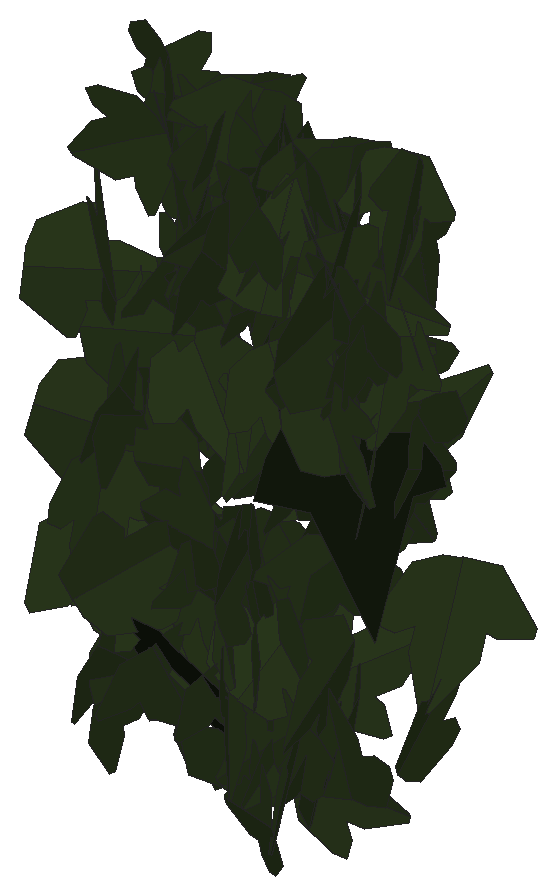
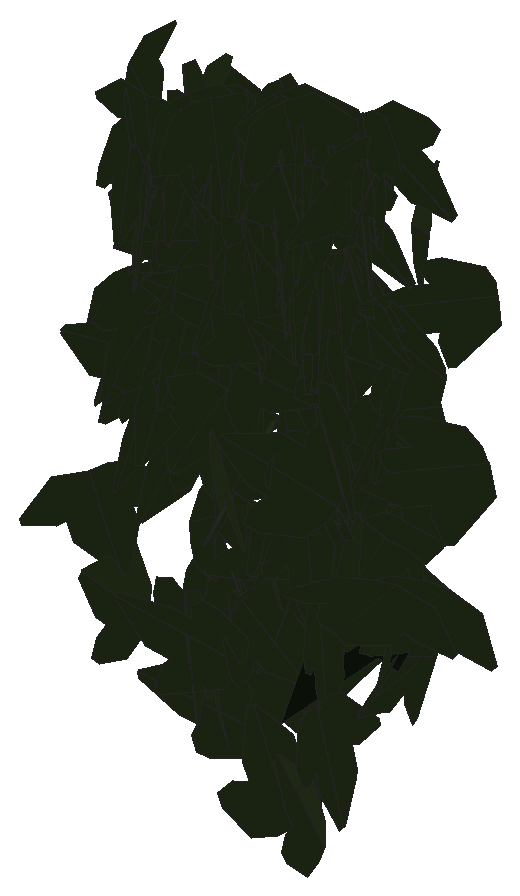
# SketchUp Ruby script. Lengths in inches.
U = 1.inch
M = Sketchup.active_model
def pt(a) = Geom::Point3d.new(a.map { |v| v * U })
def face(e, loops, mat)
  f = e.add_face(loops[0].map { |a| pt(a) })
  loops[1..].each { |l| e.add_face(l.map { |a| pt(a) }).erase! }
  f.material = f.back_material = mat if mat
  f
end
# faces: each face lists its corners as indices into pts; further lists are holes
def faces(e, pts, list, mat = nil) = list.each { |f| face(e, (f[0].is_a?(Array) ? f : [f]).map { |l| l.map { |i| pts[i] } }, mat) }
# xy, xz, yz: faces in a plane at the given z, y or x. An outline is a flat list of corners, or four numbers for a rectangle; further outlines are holes
def ring(l) = l.size == 4 ? [[l[0], l[1]], [l[2], l[1]], [l[2], l[3]], [l[0], l[3]]] : l.each_slice(2).to_a
def flat(e, list, mat, &to3) = list.each { |f| face(e, (f[0].is_a?(Array) ? f : [f]).map { |l| ring(l).map { |u, v| to3.(u, v) } }, mat) }
def xy(e, z, list, mat = nil) = flat(e, list, mat) { |x, y| [x, y, z] }
def xz(e, y, list, mat = nil) = flat(e, list, mat) { |x, z| [x, y, z] }
def yz(e, x, list, mat = nil) = flat(e, list, mat) { |y, z| [x, y, z] }
def lines(e, pts, list) = list.each { |a, b| e.add_line(pt(pts[a]), pt(pts[b])) }
# prism: a flat outline (further loops are holes) pulled along v
def prism(e, loops, v, mat = nil)
  f = face(e, loops, mat); d = Geom::Vector3d.new(v.map { |x| x * U })
  f.pushpull(f.normal.samedirection?(d) ? d.length : -d.length)
end
def box(e, o, s, mat = nil) = prism(e, [[o, [o[0] + s[0], o[1], o[2]], [o[0] + s[0], o[1] + s[1], o[2]], [o[0], o[1] + s[1], o[2]]]], [0, 0, s[2]], mat)
def at(x, y, z, deg = 0) = Geom::Transformation.translation(pt([x, y, z])) * Geom::Transformation.rotation(ORIGIN, Z_AXIS, deg.degrees)
def axes(o, x, y, z) = Geom::Transformation.new([*x, 0, *y, 0, *z, 0, *pt(o).to_a, 1])
def part(name) = M.definitions.add(name)
# library, detail: a bought-in or finely detailed component or shape, given as its bounding box
def library(name, o, s) = part(name).tap { |d| box(d.entities, o, s) }
def detail(e, o, s) = box(e.add_group.entities, o, s)
def put(e, d, t, mat = nil) = e.add_instance(d, t).tap { |i| i.material = mat if mat }
def group(e, t, mat = nil) = e.add_group.tap { |g| g.transformation = t; g.material = mat if mat }.entities
root = M.entities
M.materials.add("efeu1").color = [18, 25, 13]
M.materials.add("efeu2").color = [43, 57, 29]
c1 = part("ivyleaf_10")
p = [[0,0.5,-0.03],[-0.0625,2.02,-0.43],[-0.19,2.01,-0.46],[-0.54,1.05,-0.29],[-0.52,0.625,-0.18],[-0.83,0.76,-0.28],
  [-1.16,0.64,-0.33],[-1.15,0.33,-0.24],[-0.77,-0.39,0.02],[-0.3,-0.51,0.16],[0.04,-0.48,0.23],[-0.02,2.01,-0.4375],
  [-0.06,2.01,-0.43],[0.04,-0.49,0.23],[0.67,-0.49,0.14],[1.38,0.36,-0.2],[1.375,0.51,-0.24],[0.81,0.65,-0.19],
  [0.62,0.59,-0.15],[0.6,1.09,-0.28],[0.5,1.23,-0.31]]
faces(c1.entities,p,[[0,1,2,3,4,5,6,7,8,9,10],[11,12,0,13,14,15,16,17,18,19,20]],"efeu2")
c2 = part("ivyleaf_9")
p = [[1.54,2.16,1.25],[1.36,2.04,1.19],[-0.21,0.99,0.68],[-0.71,1.11,0.82],[-0.85,0.86,0.67],[-0.8,0.17,0.21],
  [-0.9,-0.01,0.1],[-0.67,-0.16,-0.02],[-0.08,-0.08,-0.05],[-0.03,-0.6,-0.4],[0.65,-0.88,-0.66],[0.83,-0.6,-0.49],
  [1.29,-0.42,-0.43],[1.8125,-0.07,-0.26],[1.21,0.44,0.15]]
faces(c2.entities,p,[[0,1,2,3,4,5,6,7,8,9,10,11,12,13,14]],"efeu1")
put(root,c1,axes([512.85,137.88,165.8],[-0.61365,-0.39489,-0.40861],[0.59165,-0.29438,-0.51622],[0.10906,-0.62494,0.50136]))
put(root,c1,axes([512.73,137.47,167.61],[-0.17674,-0.09364,-0.70528],[0.69487,0.13336,-0.19184],[0.15281,-0.71476,0.0566]))
put(root,c1,axes([512.85,137.07,169.74],[-0.01784,-0.10358,-0.65219],[0.5842,0.30172,-0.0639],[0.30789,-0.57848,0.08345]))
put(root,c1,axes([513.58,138.22,171.53],[0.26488,-0.35751,-0.46842],[-0.21107,0.42193,-0.44138],[0.55016,0.334,0.05618]))
put(root,c1,axes([513.83,138.29,171.4],[0.40899,-0.12558,-0.5347],[-0.49938,0.19254,-0.42719],[0.22868,0.64506,0.02342]))
put(root,c1,axes([513.6,138.05,172.16],[0.4583,-0.29069,-0.36046],[-0.16959,0.36655,-0.51122],[0.4309,0.45344,0.18218]))
put(root,c1,axes([513.5,139.38,163.08],[0.33574,-0.55507,0.20984],[-0.08731,0.19227,0.64828],[-0.58695,-0.34611,0.02359]))
put(root,c1,axes([513.97,137.29,171.7],[0.33697,-0.01814,-0.55069],[-0.52119,0.19893,-0.32547],[0.17875,0.6142,0.08915]))
put(root,c1,axes([513.6,138.19,171.47],[-0.35879,0.52593,0.01901],[-0.01059,0.01579,-0.63666],[-0.52617,-0.35895,-0.00015]))
put(root,c1,axes([513.59,137.05,167.17],[0.21935,0.60907,-0.19533],[-0.07898,-0.17912,-0.64723],[-0.63473,0.23277,0.01303]))
put(root,c1,axes([513.98,136.61,170.21],[-0.14496,0.25713,-0.65999],[-0.32484,0.57452,0.29518],[0.62943,0.35572,0.00034]))
put(root,c1,axes([513.66,137.23,168.19],[0.08621,-0.4078,-0.61317],[0.11643,0.61714,-0.39407],[0.72714,-0.05047,0.1358]))
put(root,c1,axes([513.3,138.28,165.88],[-0.64673,-0.45815,-0.35979],[0.61033,-0.38238,-0.49068],[0.10919,-0.57625,0.61165]))
put(root,c1,axes([513.76,137.1875,168.34],[-0.06088,-0.50013,-0.40046],[0.0295,0.39965,-0.5036],[0.64002,-0.066,-0.01488]))
put(root,c1,axes([513.61,138.19,171.77],[-0.03195,-0.32113,-0.5712],[0.25843,0.51935,-0.30643],[0.60216,-0.23993,0.10121]))
put(root,c1,axes([513.75,136.875,164.49],[0.11272,-0.15889,-0.69018],[0.07661,0.6975,-0.14806],[0.70408,-0.05045,0.1266]))
put(root,c1,axes([513.78,136.84,165.15],[-0.03745,-0.42888,-0.50986],[0.0562,0.50681,-0.43044],[0.66388,-0.06709,0.00768]))
put(root,c1,axes([513.86,138.65,164.04],[-0.00588,-0.63791,0.03298],[0.00167,-0.033,-0.63793],[0.63876,-0.00579,0.00197]))
put(root,c1,axes([513.27,137.51,168.89],[0.16767,-0.1235,-0.67754],[0.64533,-0.21538,0.19896],[-0.24054,-0.66391,0.06149]))
put(root,c1,axes([514.35,137.54,167.41],[-0.11672,-0.04175,0.64948],[-0.6326,-0.14775,-0.12318],[0.15291,-0.64313,-0.01386]))
put(root,c1,axes([514.07,138.37,168.32],[0.41892,-0.3409,-0.40351],[-0.26795,0.30669,-0.53728],[0.45524,0.49422,0.05508]))
put(root,c1,axes([514.4,137.75,169.58],[-0.22029,-0.00398,0.66367],[-0.66144,-0.05607,-0.21989],[0.05447,-0.69702,0.0139]))
put(root,c1,axes([514.12,138.47,170.08],[-0.54215,0.29658,0.16266],[-0.17653,0.01404,-0.61399],[-0.28854,-0.56585,0.07002]))
put(root,c1,axes([514.0625,138.02,169.72],[-0.12428,-0.64738,-0.0655],[0.00886,0.065,-0.65919],[0.65062,-0.12454,-0.00354]))
put(root,c1,axes([514.16,138.11,169.99],[-0.16882,-0.60605,-0.25],[0.07234,0.23936,-0.6291],[0.65158,-0.18359,0.00507]))
put(root,c1,axes([513.93,136.68,166.07],[-0.13402,-0.33783,0.67271],[0.23244,0.63133,0.36336],[-0.71599,0.26819,-0.00796]))
put(root,c1,axes([514.28,138.46,171.36],[-0.62156,-0.1435,0.01032],[-0.01151,0.004,-0.63788],[0.14341,-0.62163,-0.00649]))
put(root,c1,axes([514.28,138.13,165.15],[0.10717,-0.62045,-0.16683],[-0.01017,0.16748,-0.62939],[0.64241,0.10616,0.01786]))
put(root,c1,axes([513.91,138.02,168.97],[-0.05865,-0.34172,0.53698],[0.3548,0.43015,0.31248],[-0.52843,0.32674,0.15022]))
put(root,c1,axes([514.36,138.49,170.44],[0.13218,-0.58425,-0.21694],[0.00981,0.22369,-0.59645],[0.62315,0.12041,0.05541]))
put(root,c1,axes([514.38,137.72,170.74],[0.50532,-0.40252,-0.09325],[-0.06531,0.06764,-0.64593],[0.40798,0.50938,0.01209]))
put(root,c1,axes([514.09,138.6,167.28],[-0.13344,-0.43712,0.49629],[0.28939,0.41665,0.44479],[-0.59467,0.30085,0.10509]))
put(root,c1,axes([514.375,137.11,165.08],[-0.27121,-0.5559,-0.2919],[0.13254,0.26012,-0.61851],[0.61373,-0.30183,0.00458]))
put(root,c1,axes([514.33,138.89,162.96],[-0.17352,-0.63394,0.08937],[0.0274,0.08516,0.65725],[-0.63962,0.17563,0.00391]))
put(root,c2,axes([514.18,137.0625,165.29],[0.7452,0.01057,-0.14491],[-0.14507,0.01144,-0.74516],[-0.00819,0.75908,0.01325]))
put(root,c1,axes([514.4,137.58,171.39],[-0.21766,0.6227,0.01951],[-0.00888,0.01756,-0.65964],[-0.62294,-0.21783,0.00259]))
put(root,c1,axes([514.13,137.29,165.84],[0.54414,0.22993,0.3502],[0.31112,0.16265,-0.5902],[-0.28056,0.62631,0.02471]))
put(root,c1,axes([514.5,137.49,166.12],[-0.56081,0.34214,-0.00262],[0.00161,-0.00238,-0.65694],[-0.34214,-0.56081,0.00119]))
put(root,c1,axes([514.53,138.13,171.75],[0.19232,-0.6045,-0.13853],[0.03492,0.15536,-0.62948],[0.61919,0.179,0.07853]))
put(root,c1,axes([514.52,138.26,167.42],[-0.05116,-0.50073,-0.41595],[0.0861,0.40837,-0.50219],[0.64524,-0.09419,0.03403]))
put(root,c1,axes([515.03,137.06,166.9],[-0.08013,0.00077,0.65378],[-0.65112,0.05918,-0.07987],[-0.05883,-0.656,-0.00643]))
put(root,c1,axes([514.48,137.93,171.34],[0.07676,-0.47822,0.43051],[0.21187,-0.3906,-0.47166],[0.60757,0.19663,0.11009]))
put(root,c1,axes([514.69,138.3,172.05],[-0.30495,-0.55748,0.12489],[0.00644,-0.14492,-0.63113],[0.57126,-0.29596,0.07379]))
put(root,c1,axes([514.56,138.44,171.42],[0.38938,-0.48932,0.14193],[0.08873,-0.11077,-0.62534],[0.5017,0.39936,0.00045]))
put(root,c1,axes([514.72,138.41,170.64],[0.25734,-0.56848,-0.14836],[-0.00045,0.16178,-0.62067],[0.58752,0.24912,0.0645]))
put(root,c1,axes([514.92,138.125,172.03],[-0.41926,-0.40959,0.25796],[-0.07906,-0.27875,-0.57109],[0.47756,-0.40574,0.13193]))
put(root,c1,axes([514.86,137.73,166.19],[-0.22876,-0.6235,-0.0101],[0.00452,0.0091,-0.66414],[0.62356,-0.22881,0.00111]))
put(root,c1,axes([515.07,138.4375,171.2],[-0.16129,-0.60038,0.14721],[-0.01655,-0.14788,-0.62129],[0.61794,-0.16067,0.02178]))
put(root,c1,axes([514.6875,137.42,168.93],[0.52805,0.24001,0.31496],[0.28358,0.1372,-0.58],[-0.27638,0.59934,0.00665]))
put(root,c1,axes([515.01,138.02,171.85],[-0.03878,0.49339,0.40523],[-0.10112,0.3961,-0.49196],[-0.63041,-0.09389,0.05398]))
put(root,c1,axes([515.14,138.46,170.15],[-0.02485,-0.6374,-0.01661],[-0.00182,0.01669,-0.63788],[0.63762,-0.0248,-0.00246]))
put(root,c1,axes([515.125,137.73,170.91],[-0.05733,0.00792,-0.69212],[-0.17006,-0.67336,0.00639],[-0.67095,0.17,0.05752]))
put(root,c1,axes([515.09,137.49,166.67],[-0.4488,-0.41114,-0.31279],[0.22186,0.22078,-0.60854],[0.46653,-0.50051,-0.0115]))
put(root,c1,axes([514.73,137.41,166.33],[0.45052,-0.16717,0.56701],[0.54609,-0.15526,-0.47968],[0.22633,0.70736,0.02871]))
put(root,c1,axes([515.23,138.33,171.35],[0.03482,-0.62539,-0.12878],[0.0028,0.12912,-0.62629],[0.63851,0.03354,0.00977]))
put(root,c1,axes([515.24,138.1,171.66],[0.18577,-0.58758,-0.16925],[0.00891,0.17947,-0.61328],[0.6114,0.17591,0.06036]))
put(root,c1,axes([515.27,138.22,164.91],[-0.14679,-0.50179,0.37147],[0.0513,-0.39,-0.50655],[0.62221,-0.08622,0.1294]))
put(root,c1,axes([515.14,137.63,166.29],[-0.61598,0.16189,0.30669],[0.29357,-0.08938,0.63681],[0.18462,0.68228,0.01065]))
put(root,c1,axes([515.25,137.21,165.14],[-0.21552,-0.48565,-0.40585],[0.18304,0.36258,-0.53108],[0.60586,-0.2823,0.01608]))
put(root,c1,axes([515.3,138.2,168.33],[-0.16799,-0.36698,0.51188],[0.11684,-0.53874,-0.34789],[0.61891,0.0021,0.20462]))
put(root,c1,axes([515.375,137.79,170.16],[0.03622,-0.59354,-0.25176],[0.02959,0.25342,-0.5932],[0.64405,0.02174,0.04141]))
put(root,c1,axes([515.42,136.65,170.94],[-0.00724,-0.47935,-0.49437],[0.03839,0.49334,-0.47892],[0.68753,-0.03259,0.02154]))
put(root,c1,axes([515.19,137.54,163.7],[-0.42781,-0.42933,0.34425],[0.26159,0.22496,0.60565],[-0.48415,0.50092,0.02305]))
put(root,c1,axes([515.53,137.92,169.53],[0.20746,-0.57715,-0.18427],[-0.03543,0.18289,-0.61269],[0.60482,0.20868,0.02732]))
put(root,c1,axes([515.82,137.01,171.4],[-0.47564,0.162,0.39647],[-0.41372,-0.02057,-0.48794],[-0.11076,-0.61887,0.12]))
put(root,c1,axes([515.54,137.4,169],[0.26815,-0.36345,0.57601],[-0.23798,0.53003,0.44522],[-0.63816,-0.35037,0.076]))
put(root,c1,axes([515.32,137.25,165.11],[-0.15294,0.53976,-0.39567],[0.11258,-0.37934,-0.56099],[-0.65971,-0.18986,-0.00401]))
put(root,c1,axes([515.96,137.07,163.53],[-0.1417,0.05142,0.62374],[-0.59714,0.18037,-0.15053],[-0.18738,-0.61367,0.00802]))
put(root,c1,axes([515.78,136.6,166.65],[-0.00549,-0.01778,0.68873],[-0.4264,0.54108,0.01057],[-0.54116,-0.42616,-0.01531]))
put(root,c1,axes([516.03,137.43,164.55],[-0.45792,-0.06403,0.53508],[-0.51627,-0.14922,-0.45968],[0.15452,-0.68828,0.04988]))
put(root,c1,axes([515.3,137.75,165.53],[0.0449,-0.11336,0.64522],[0.48975,-0.42372,-0.10853],[0.43509,0.48865,0.05557]))
put(root,c1,axes([515.78,137.93,171.69],[-0.53871,0.31995,0.11542],[-0.12896,0.00792,-0.62386],[-0.31474,-0.55088,0.05806]))
put(root,c1,axes([515.4,137.7,169.84],[0.33476,-0.3555,-0.47492],[0.33213,-0.33953,0.48826],[-0.49155,-0.47152,0.00647]))
put(root,c1,axes([515.79,137.99,164.39],[0.07036,0.32415,-0.55107],[-0.11991,-0.53787,-0.3317],[-0.628,0.13902,0.00159]))
put(root,c1,axes([516.11,137.59,169.7],[0.50092,0.00863,0.51223],[-0.50939,0.08467,0.49672],[-0.05455,-0.71143,0.06533]))
put(root,c1,axes([515.83,137.88,169.6],[0.04992,-0.38401,-0.51185],[0.06174,0.5139,-0.37953],[0.6369,-0.01972,0.07691]))
put(root,c1,axes([515.33,138.34,169.2],[-0.07088,-0.19303,0.65615],[0.60537,0.28929,0.1505],[-0.3183,0.59318,0.14012]))
put(root,c1,axes([515.83,137.63,170.7],[-0.20664,-0.53988,-0.30294],[0.13466,0.27252,-0.57753],[0.60424,-0.24536,0.02511]))
put(root,c1,axes([515.93,138.25,171.65],[-0.39204,-0.51318,0.08154],[0.03388,-0.12718,-0.63748],[0.51851,-0.3797,0.10331]))
put(root,c1,axes([515.91,138.0625,166.99],[0.22098,-0.60664,-0.00253],[-0.00087,0.00238,-0.64563],[0.60665,0.22098,-0.00001]))
put(root,c1,axes([515.78,137.29,170.42],[0.49325,0.3722,-0.16877],[0.13694,0.09872,0.61791],[0.38506,-0.51189,-0.00355]))
put(root,c1,axes([515.66,137.25,165.28],[0.5017,0.21544,-0.38775],[0.32517,0.21954,0.54271],[0.30171,-0.59486,0.05986]))
put(root,c1,axes([516.05,137.99,164.1875],[0.15354,-0.61507,-0.08584],[-0.0151,0.0847,-0.63392],[0.62085,0.15417,0.00581]))
put(root,c1,axes([515.54,138.73,164.57],[0.32504,0.02522,-0.59187],[0.57766,0.1362,0.32304],[0.13135,-0.66137,0.04396]))
put(root,c1,axes([516.1,137.21,166.46],[0.31977,-0.19965,-0.61096],[0.00723,0.68347,-0.21956],[0.64272,0.09165,0.30644]))
put(root,c1,axes([516.18,138.3,171.65],[-0.25248,-0.59193,0.08358],[0.01803,-0.09823,-0.64121],[0.59753,-0.24715,0.05466]))
put(root,c1,axes([515.87,138.23,167.75],[0.45126,0.33707,0.3113],[0.25941,0.17273,-0.56306],[-0.37846,0.5203,-0.01475]))
put(root,c1,axes([516.27,138.23,164.58],[0.22996,-0.53729,-0.27231],[-0.08288,0.26049,-0.58395],[0.59663,0.24327,0.02384]))
put(root,c1,axes([516.27,137.49,168.16],[-0.01388,-0.57456,-0.32341],[0.00142,0.32345,-0.5747],[0.65933,-0.01279,-0.00557]))
put(root,c1,axes([515.72,138.23,163.44],[-0.05873,-0.04999,0.68185],[0.66965,0.13374,0.06749],[-0.13781,0.67118,0.03734]))
put(root,c1,axes([516.14,137.375,164.67],[0.4345,-0.46873,0.30165],[0.20045,-0.22549,-0.63911],[0.52011,0.47847,-0.00569]))
put(root,c1,axes([516.19,137.59,169.34],[0.01159,-0.16452,-0.62767],[0.02812,-0.62705,0.16488],[-0.64826,-0.03014,-0.00407]))
put(root,c1,axes([516.41,137.57,169.34],[-0.02473,0.03408,0.67814],[-0.22507,0.63981,-0.04036],[-0.64061,-0.2261,-0.01199]))
put(root,c1,axes([516.17,136.98,169.54],[0.36435,0.51118,0.17961],[0.0816,0.1622,-0.62718],[-0.53564,0.37242,0.02663]))
put(root,c1,axes([516.44,137.64,166.9],[-0.24329,-0.56355,0.17761],[0.00176,-0.19277,-0.60923],[0.59088,-0.23147,0.07494]))
put(root,c1,axes([516.36,137.98,168.77],[-0.14984,-0.53214,-0.32558],[0.14705,0.29527,-0.55029],[0.60626,-0.20314,0.05301]))
put(root,c1,axes([516.46,138.03,170.99],[-0.56623,0.29359,-0.00032],[0.00048,0.00023,-0.63782],[-0.29359,-0.56623,-0.00042]))
put(root,c1,axes([516.58,137.71,164.01],[-0.66682,-0.09016,-0.06399],[-0.06233,-0.01655,0.67284],[-0.09131,0.66968,0.00801]))
put(root,c1,axes([516.5,138.3,168.26],[-0.27107,-0.58819,-0.26203],[0.13452,0.22631,-0.64715],[0.62971,-0.30154,0.02544]))
put(root,c1,axes([516.28,137.37,169.55],[0.04361,-0.11778,0.71708],[0.37618,0.61829,0.07868],[-0.62175,0.36583,0.0979]))
put(root,c1,axes([516.53,137.6,165.58],[0.02746,-0.20104,0.6447],[0.27965,-0.58393,-0.194],[0.6147,0.27464,0.05946]))
put(root,c1,axes([516.76,137.65,171.55],[0.2716,-0.55572,-0.21183],[-0.04667,0.21224,-0.61663],[0.59289,0.27128,0.04849]))
put(root,c1,axes([516.65,138.5,168.99],[-0.29508,-0.48275,-0.34445],[0.20228,0.27973,-0.56533],[0.55747,-0.35703,0.02281]))
put(root,c1,axes([517.11,136.89,170.86],[-0.09071,0.19805,-0.6082],[-0.41302,0.45091,0.20843],[0.4884,0.4181,0.0633]))
put(root,c1,axes([516.71,137.69,166.91],[-0.25282,-0.46382,-0.38639],[0.17549,0.34435,-0.52818],[0.5776,-0.30763,-0.00865]))
put(root,c1,axes([516.78,138.33,167.67],[0.01121,-0.53491,-0.37796],[0.12939,0.37237,-0.52317],[0.64206,-0.0657,0.11203]))
put(root,c1,axes([516.93,137.6,168.35],[0.42317,-0.44683,-0.21759],[-0.13813,0.16877,-0.61523],[0.47741,0.4449,0.01486]))
put(root,c1,axes([516.93,137.08,168.83],[0.03239,0.65673,-0.17983],[-0.00395,0.18021,0.65741],[0.68089,-0.03019,0.01236]))
put(root,c1,axes([516.98,136.4,170.27],[0.08915,-0.12975,0.77518],[-0.26672,0.72886,0.15267],[-0.73933,-0.27859,0.03839]))
put(root,c1,axes([517.13,138.14,170.3125],[-0.3309,0.32557,0.43627],[-0.33746,0.27793,-0.46336],[-0.42714,-0.47179,0.0281]))
put(root,c1,axes([517.27,137.16,170.625],[-0.52627,-0.00248,0.43532],[-0.43531,0.00979,-0.52619],[-0.00433,-0.68291,-0.00912]))
put(root,c1,axes([516.71,137.1,169.23],[-0.53467,0.16729,-0.30873],[0.29059,-0.10493,-0.56011],[-0.19713,-0.60842,0.01171]))
put(root,c1,axes([516.77,138.43,171.64],[0.62939,0.04433,0.095],[0.09595,-0.01054,-0.63072],[-0.04225,0.63644,-0.01706]))
put(root,c1,axes([517.02,137.5,169.96],[-0.00918,-0.54484,-0.35414],[0.08233,0.35035,-0.54114],[0.64459,-0.05251,0.06407]))
put(root,c1,axes([516.54,137.43,170.58],[0.13342,0.0934,0.70297],[0.53369,0.4578,-0.16212],[-0.46697,0.54989,0.01557]))
put(root,c1,axes([516.76,138.29,168.12],[0.21058,0.25817,-0.65257],[0.40139,0.51456,0.3331],[0.57566,-0.45323,0.00646]))
put(root,c1,axes([517.08,138.36,171.06],[-0.04769,-0.61268,-0.18724],[0.0886,0.17965,-0.6104],[0.6345,-0.07114,0.07116]))
put(root,c1,axes([517.24,138.18,168.76],[-0.25429,-0.62194,0.03039],[-0.01117,-0.02826,-0.67192],[0.62258,-0.25453,0.00035]))
put(root,c2,axes([516.92,137.48,168.72],[-0.08579,-0.76793,-0.21996],[0.04423,0.21632,-0.77247],[0.79759,-0.0946,0.01918]))
put(root,c1,axes([517.2,138.29,164.39],[0.20728,-0.47978,0.46203],[-0.15792,0.43469,0.52224],[-0.64709,-0.25977,0.02055]))
put(root,c1,axes([517.1,137.84,169.9],[0.64732,-0.0105,0.03973],[0.03978,0.00237,-0.64739],[0.01033,0.64853,0.003]))
put(root,c1,axes([517.19,137.43,170.24],[0.06673,-0.4912,-0.42817],[0.09597,0.43312,-0.48192],[0.64451,-0.01363,0.11609]))
put(root,c1,axes([517.42,137.92,168.32],[0.05905,-0.33084,-0.56657],[-0.00445,0.56865,-0.33252],[0.65608,0.03363,0.04874]))
put(root,c1,axes([517.1875,138.125,171.83],[0.09119,-0.47855,0.4245],[0.29353,-0.34968,-0.45726],[0.56838,0.25737,0.16804]))
put(root,c1,axes([517.34,138.79,166.29],[0.51087,0.48886,-0.15534],[-0.11096,-0.10872,-0.70708],[-0.5008,0.52278,-0.00179]))
